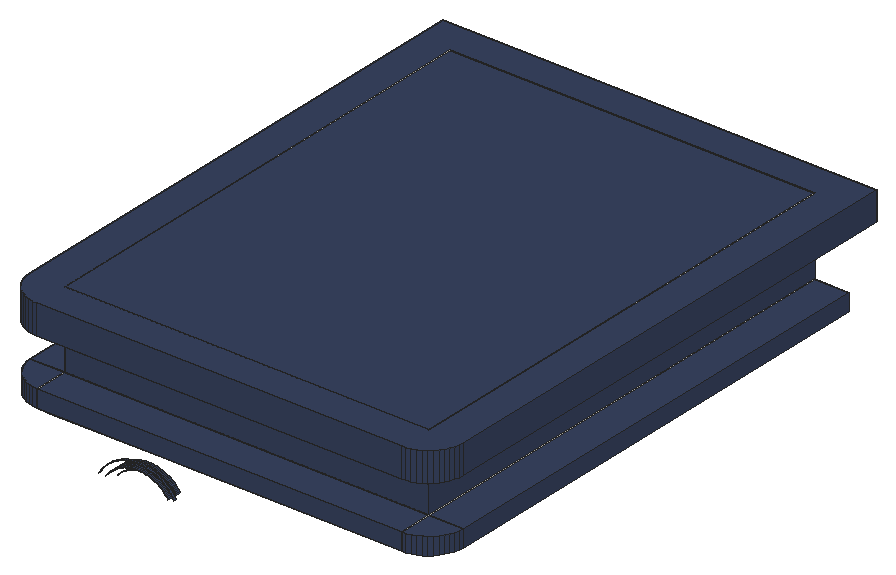
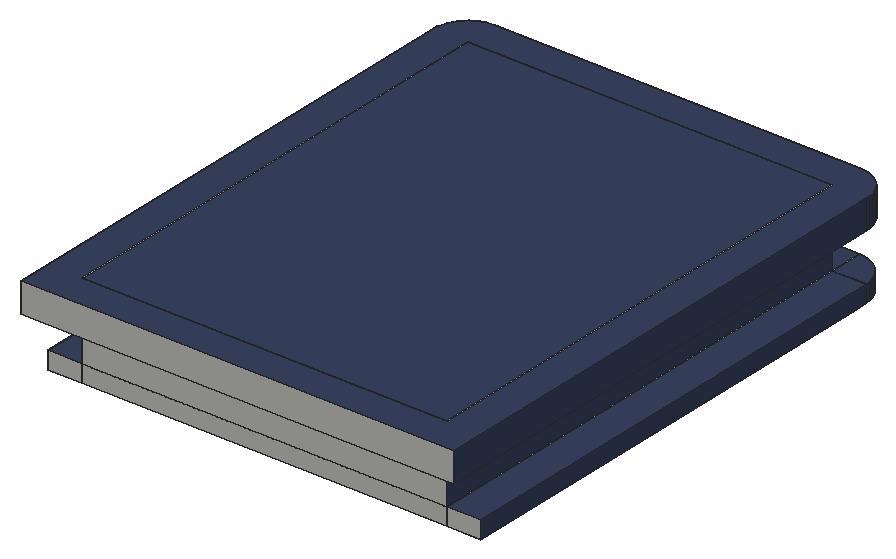
# SketchUp Ruby script. Lengths in inches.
U = 1.inch
M = Sketchup.active_model
def pt(a) = Geom::Point3d.new(a.map { |v| v * U })
def face(e, loops, mat)
  f = e.add_face(loops[0].map { |a| pt(a) })
  loops[1..].each { |l| e.add_face(l.map { |a| pt(a) }).erase! }
  f.material = f.back_material = mat if mat
  f
end
# faces: each face lists its corners as indices into pts; further lists are holes
def faces(e, pts, list, mat = nil) = list.each { |f| face(e, (f[0].is_a?(Array) ? f : [f]).map { |l| l.map { |i| pts[i] } }, mat) }
# xy, xz, yz: faces in a plane at the given z, y or x. An outline is a flat list of corners, or four numbers for a rectangle; further outlines are holes
def ring(l) = l.size == 4 ? [[l[0], l[1]], [l[2], l[1]], [l[2], l[3]], [l[0], l[3]]] : l.each_slice(2).to_a
def flat(e, list, mat, &to3) = list.each { |f| face(e, (f[0].is_a?(Array) ? f : [f]).map { |l| ring(l).map { |u, v| to3.(u, v) } }, mat) }
def xy(e, z, list, mat = nil) = flat(e, list, mat) { |x, y| [x, y, z] }
def xz(e, y, list, mat = nil) = flat(e, list, mat) { |x, z| [x, y, z] }
def yz(e, x, list, mat = nil) = flat(e, list, mat) { |y, z| [x, y, z] }
def lines(e, pts, list) = list.each { |a, b| e.add_line(pt(pts[a]), pt(pts[b])) }
# prism: a flat outline (further loops are holes) pulled along v
def prism(e, loops, v, mat = nil)
  f = face(e, loops, mat); d = Geom::Vector3d.new(v.map { |x| x * U })
  f.pushpull(f.normal.samedirection?(d) ? d.length : -d.length)
end
def box(e, o, s, mat = nil) = prism(e, [[o, [o[0] + s[0], o[1], o[2]], [o[0] + s[0], o[1] + s[1], o[2]], [o[0], o[1] + s[1], o[2]]]], [0, 0, s[2]], mat)
def at(x, y, z, deg = 0) = Geom::Transformation.translation(pt([x, y, z])) * Geom::Transformation.rotation(ORIGIN, Z_AXIS, deg.degrees)
def axes(o, x, y, z) = Geom::Transformation.new([*x, 0, *y, 0, *z, 0, *pt(o).to_a, 1])
def part(name) = M.definitions.add(name)
# library, detail: a bought-in or finely detailed component or shape, given as its bounding box
def library(name, o, s) = part(name).tap { |d| box(d.entities, o, s) }
def detail(e, o, s) = box(e.add_group.entities, o, s)
def put(e, d, t, mat = nil) = e.add_instance(d, t).tap { |i| i.material = mat if mat }
def group(e, t, mat = nil) = e.add_group.tap { |g| g.transformation = t; g.material = mat if mat }.entities
root = M.entities
M.materials.add("0360 AP 9644 Monsoon Midnight-N").color = [56, 67, 95]
M.materials.add("[Color M07]").color = [58, 58, 58]
xy(root,360,[[24,89.9375,33,98.79],[33,89.9375,117.8125,98.79],[117.8125,89.9375,126.8125,425.9375],[0,98.79,24,98.9375],[24,98.79,33,98.9375],
  [24,98.9375,33,425.9375],[126.8125,125.9375,269.3125,134.9375],[269.3125,125.9375,278.3125,134.9375],[126.8125,134.9375,269.3125,417.55],[269.3125,134.9375,278.3125,425.9375],
  [33,416.9375,117.8125,425.9375],[126.8125,417.55,269.3125,425.9375]])
xy(root,360,[[24,65.9375,20.95,66.36,17.98,67.14,15.12,68.27,12.4,69.72,9.88,71.48,7.58,73.52,5.54,75.82,3.78,78.34,2.33,81.05,1.21,83.92,0.43,86.89,0,89.9375,24,89.9375],[24,65.9375,33,89.9375],[33,65.9375,117.8125,89.9375],[117.8125,65.9375,126.8125,89.9375],[126.8125,65.9375,269.3125,89.9375],
  [269.3125,65.9375,278.3125,89.9375],[278.3125,65.9375,278.3125,89.9375,302.3125,89.9375,302.02,86.84,301.34,83.8,300.28,80.875,298.87,78.1,297.12,75.53,295.06,73.19,292.72,71.13,290.15,69.38,287.375,67.97,284.45,66.91,281.41,66.23],[0,89.9375,24,98.79],[126.8125,89.9375,269.3125,125.9375],[269.3125,89.9375,278.3125,125.9375],
  [278.3125,89.9375,302.3125,125.9375],[33,98.79,117.8125,416.9375],[0,98.9375,24,425.9375],[278.3125,125.9375,302.3125,134.9375],[278.3125,134.9375,302.3125,425.9375]],"0360 AP 9644 Monsoon Midnight-N")
xy(root,372,[[24,89.9375,278.3125,425.9375]])
xy(root,372,[[24,65.9375,24,89.9375,0,89.9375,0.43,86.89,1.21,83.92,2.33,81.05,3.78,78.34,5.54,75.82,7.58,73.52,9.88,71.48,12.4,69.72,15.12,68.27,17.98,67.14,20.95,66.36],[24,65.9375,278.3125,89.9375],[278.3125,65.9375,281.41,66.23,284.45,66.91,287.375,67.97,290.15,69.38,292.72,71.13,295.06,73.19,297.12,75.53,298.87,78.1,300.28,80.875,301.34,83.8,302.02,86.84,302.3125,89.9375,278.3125,89.9375],[0,89.9375,24,425.9375],[278.3125,89.9375,302.3125,425.9375]],"0360 AP 9644 Monsoon Midnight-N")
xy(root,405.375,[[24,89.9375,278.3125,425.9375]])
xy(root,405.375,[[[24,65.9375,20.87,66.14,17.79,66.76,14.82,67.76,12,69.15,9.39,70.9,7.03,72.97,4.96,75.33,3.22,77.9375,1.83,80.75,0.82,83.73,0.21,86.8,0,89.9375,0,449.9375,302.3125,449.9375,302.3125,89.9375,302.11,86.8,301.49,83.73,300.49,80.75,299.1,77.9375,297.35,75.33,295.28,72.97,292.92,70.9,290.3125,69.15,287.5,67.76,284.52,66.76,281.45,66.14,278.3125,65.9375],[24,89.9375,278.3125,425.9375]]],"0360 AP 9644 Monsoon Midnight-N")
xy(root,425.625,[[[24,65.9375,278.3125,65.9375,281.45,66.14,284.52,66.76,287.5,67.76,290.3125,69.15,292.92,70.9,295.28,72.97,297.35,75.33,299.1,77.9375,300.49,80.75,301.49,83.73,302.11,86.8,302.3125,89.9375,302.3125,449.9375,0,449.9375,0,89.9375,0.21,86.8,0.82,83.73,1.83,80.75,3.22,77.9375,4.96,75.33,7.03,72.97,9.39,70.9,12,69.15,14.82,67.76,17.79,66.76,20.87,66.14],[24,89.9375,278.3125,425.9375]],[24,89.9375,278.3125,425.9375]],"0360 AP 9644 Monsoon Midnight-N")
xz(root,65.9375,[[24,360,278.3125,372],[24,405.375,278.3125,425.625]],"0360 AP 9644 Monsoon Midnight-N")
xz(root,89.9375,[[0,360,24,372],[24,360,278.3125,372],[278.3125,360,302.3125,372],[24,405.375,278.3125,425.625]])
xz(root,89.9375,[[24,372,278.3125,405.375]],"0360 AP 9644 Monsoon Midnight-N")
xz(root,425.9375,[[0,360,24,372],[24,360,278.3125,372],[278.3125,360,302.3125,372],[24,372,278.3125,405.375],[24,405.375,278.3125,425.625]])
xz(root,449.9375,[[0,405.375,302.3125,425.625]])
yz(root,0,[[89.9375,360,425.9375,372],[89.9375,405.375,449.9375,425.625]],"0360 AP 9644 Monsoon Midnight-N")
yz(root,24,[[65.9375,360,89.9375,372],[89.9375,360,425.9375,372],[89.9375,405.375,425.9375,425.625]])
yz(root,24,[[89.9375,372,425.9375,405.375]],"0360 AP 9644 Monsoon Midnight-N")
yz(root,278.3125,[[65.9375,360,89.9375,372],[89.9375,360,425.9375,372],[89.9375,405.375,425.9375,425.625]])
yz(root,278.3125,[[89.9375,372,425.9375,405.375]],"0360 AP 9644 Monsoon Midnight-N")
yz(root,302.3125,[[89.9375,360,425.9375,372],[89.9375,405.375,449.9375,425.625]],"0360 AP 9644 Monsoon Midnight-N")
p = [[49.86,89.9375,319.39],[49.35,89.9375,318.51],[49.35,88.375,318.51],[49.86,88.375,319.39],[58.67,94.27,318.47],[59.18,94.27,319.04],
  [59.18,93.58,319.04],[58.67,93.58,318.47],[92.95,94.27,319.04],[93.45,94.27,318.47],[93.45,93.58,318.47],[92.95,93.58,319.04],
  [92.95,94.96,319.04],[93.45,94.96,318.47],[54.4,88.375,318.69],[54.4,93.58,318.69],[54.91,93.58,319.4],[54.91,88.375,319.4],
  [97.21,88.375,319.4],[97.21,93.58,319.4],[97.73,93.58,318.69],[97.73,88.375,318.69],[54.91,94.96,319.4],[54.4,94.96,318.69],
  [97.73,94.96,318.69],[97.21,94.96,319.4],[54.91,98.79,319.4],[54.4,98.79,318.69],[97.73,98.79,318.69],[97.21,98.79,319.4],
  [59.7,94.27,319.59],[59.7,93.58,319.59],[92.42,94.27,319.59],[92.42,93.58,319.59],[92.42,94.96,319.59],[50.4,89.9375,320.25],
  [50.4,88.375,320.25],[55.45,93.58,320.09],[55.45,88.375,320.09],[96.68,88.375,320.09],[96.68,93.58,320.09],[55.45,94.96,320.09],
  [96.68,94.96,320.09],[55.45,98.79,320.09],[96.68,98.79,320.09],[60.24,94.27,320.125],[60.24,93.58,320.125],[91.88,94.27,320.125],
  [91.88,93.58,320.125],[91.88,94.96,320.125],[101.93,89.9375,319.69],[100.8,89.9375,321.43],[100.8,88.375,321.43],[101.93,88.375,319.69],
  [56.01,93.58,320.76],[56.01,88.375,320.76],[96.12,88.375,320.76],[96.12,93.58,320.76],[56.01,94.96,320.76],[60.8,94.27,320.64],
  [60.8,93.58,320.64],[91.32,94.27,320.64],[91.32,93.58,320.64],[96.12,94.96,320.76],[91.32,94.96,320.64],[56.01,98.79,320.76],
  [96.12,98.79,320.76],[50.97,89.9375,321.09],[50.97,88.375,321.09],[61.375,94.27,321.13],[61.375,93.58,321.13],[90.75,94.27,321.13],
  [90.75,93.58,321.13],[90.75,94.96,321.13],[56.59,93.58,321.42],[56.59,88.375,321.42],[95.54,88.375,321.42],[95.54,93.58,321.42],
  [56.59,94.96,321.42],[95.54,94.96,321.42],[56.59,98.79,321.42],[95.54,98.79,321.42],[51.57,89.9375,321.91],[51.57,88.375,321.91],
  [61.97,94.27,321.61],[61.97,93.58,321.61],[90.16,94.27,321.61],[90.16,93.58,321.61],[90.16,94.96,321.61],[57.19,93.58,322.05],
  [57.19,88.375,322.05],[94.93,88.375,322.05],[94.93,93.58,322.05],[99.56,89.9375,323.08],[99.56,88.375,323.08],[57.19,94.96,322.05],
  [94.93,94.96,322.05],[57.19,98.79,322.05],[94.93,98.79,322.05],[62.57,94.27,322.07],[62.57,93.58,322.07],[89.55,94.27,322.07],
  [89.55,93.58,322.07],[89.55,94.96,322.07],[52.1875,89.9375,322.71],[52.1875,88.375,322.71],[57.81,93.58,322.67],[57.81,88.375,322.67],
  [94.31,88.375,322.67],[94.31,93.58,322.67],[57.81,94.96,322.67],[63.19,94.27,322.51],[63.19,93.58,322.51],[88.93,94.27,322.51],
  [88.93,93.58,322.51],[94.31,94.96,322.67],[88.93,94.96,322.51],[57.81,98.79,322.67],[94.31,98.79,322.67],[63.83,94.27,322.92],
  [63.83,93.58,322.92],[88.3,94.27,322.92],[88.3,93.58,322.92],[88.3,94.96,322.92],[52.84,89.9375,323.49],[52.84,88.375,323.49],
  [58.46,93.58,323.26],[58.46,88.375,323.26],[93.67,88.375,323.26],[93.67,93.58,323.26],[58.46,94.96,323.26],[93.67,94.96,323.26],
  [58.46,98.79,323.26],[93.67,98.79,323.26],[64.48,94.27,323.32],[64.48,93.58,323.32],[87.65,94.27,323.32],[87.65,93.58,323.32],
  [87.65,94.96,323.32],[98.23,89.9375,324.66],[98.23,88.375,324.66],[59.12,93.58,323.84],[59.12,88.375,323.84],[93,88.375,323.84],
  [93,93.58,323.84],[59.12,94.96,323.84],[65.14,94.27,323.6875],[65.14,93.58,323.6875],[86.99,94.27,323.6875],[86.99,93.58,323.6875],
  [93,94.96,323.84],[86.99,94.96,323.6875],[59.12,98.79,323.84],[93,98.79,323.84],[53.51,89.9375,324.25],[53.51,88.375,324.25],
  [65.8125,94.27,324.04],[65.8125,93.58,324.04],[86.3125,94.27,324.04],[86.3125,93.58,324.04],[86.3125,94.96,324.04],[59.8,93.58,324.39],
  [59.8,88.375,324.39],[92.32,88.375,324.39],[92.32,93.58,324.39],[59.8,94.96,324.39],[92.32,94.96,324.39],[59.8,98.79,324.39],
  [92.32,98.79,324.39],[66.5,94.27,324.37],[66.5,93.58,324.37],[85.63,94.27,324.37],[85.63,93.58,324.37],[85.63,94.96,324.37],
  [54.21,89.9375,324.98],[54.21,88.375,324.98],[60.5,93.58,324.91],[60.5,88.375,324.91],[91.625,88.375,324.91],[91.625,93.58,324.91],
  [60.5,94.96,324.91],[67.19,94.27,324.67],[67.19,93.58,324.67],[84.93,94.27,324.67],[84.93,93.58,324.67],[91.625,94.96,324.91],
  [84.93,94.96,324.67],[60.5,98.79,324.91],[91.625,98.79,324.91],[97.92,89.9375,324.98],[97.92,88.375,324.98],[67.9,94.27,324.95],
  [67.9,93.58,324.95],[84.23,94.27,324.95],[84.23,93.58,324.95],[84.23,94.96,324.95],[61.22,93.58,325.42],[61.22,88.375,325.42],
  [90.91,88.375,325.42],[90.91,93.58,325.42],[61.22,94.96,325.42],[90.91,94.96,325.42],[61.22,98.79,325.42],[90.91,98.79,325.42],
  [54.93,89.9375,325.7],[54.93,88.375,325.7],[97.2,89.9375,325.7],[97.2,88.375,325.7],[68.61,94.27,325.21],[68.61,93.58,325.21],
  [83.52,94.27,325.21],[83.52,93.58,325.21],[83.52,94.96,325.21],[69.33,94.27,325.45],[69.33,93.58,325.45],[82.79,94.27,325.45],
  [82.79,93.58,325.45],[82.79,94.96,325.45],[61.95,93.58,325.9],[61.95,88.375,325.9],[90.17,88.375,325.9],[90.17,93.58,325.9],
  [61.95,94.96,325.9],[70.06,94.27,325.66],[70.06,93.58,325.66],[82.06,94.27,325.66],[82.06,93.58,325.66],[90.17,94.96,325.9],
  [82.06,94.96,325.66],[61.95,98.79,325.9],[90.17,98.79,325.9],[55.67,89.9375,326.38],[55.67,88.375,326.38],[96.45,89.9375,326.38],
  [96.45,88.375,326.38],[70.8,94.27,325.85],[70.8,93.58,325.85],[81.33,94.27,325.85],[81.33,93.58,325.85],[81.33,94.96,325.85],
  [71.54,94.27,326.01],[71.54,93.58,326.01],[80.59,94.27,326.01],[80.59,93.58,326.01],[80.59,94.96,326.01],[62.7,93.58,326.35],
  [62.7,88.375,326.35],[89.43,88.375,326.35],[89.43,93.58,326.35],[62.7,94.96,326.35],[89.43,94.96,326.35],[62.7,98.79,326.35],
  [89.43,98.79,326.35],[72.28,94.27,326.15],[72.28,93.58,326.15],[79.84,94.27,326.15],[79.84,93.58,326.15],[79.84,94.96,326.15],
  [73.03,94.27,326.26],[73.03,93.58,326.26],[79.09,94.27,326.26],[79.09,93.58,326.26],[79.09,94.96,326.26],[73.03,94.96,326.26],
  [73.79,94.96,326.35],[73.79,93.58,326.35],[74.55,94.96,326.41],[74.55,93.58,326.41],[77.58,94.27,326.41],[78.34,94.27,326.35],
  [78.34,93.58,326.35],[77.58,93.58,326.41],[77.58,94.96,326.41],[78.34,94.96,326.35],[56.44,89.9375,327.05],[56.44,88.375,327.05],
  [63.46,93.58,326.78],[63.46,88.375,326.78],[88.66,88.375,326.78],[88.66,93.58,326.78],[95.68,89.9375,327.05],[95.68,88.375,327.05],
  [63.46,94.96,326.78],[75.3,94.96,326.45],[75.3,93.58,326.45],[76.0625,94.96,326.46],[76.0625,94.27,326.46],[76.0625,93.58,326.46],
  [76.82,94.27,326.45],[76.82,93.58,326.45],[88.66,94.96,326.78],[76.82,94.96,326.45],[63.46,98.79,326.78],[88.66,98.79,326.78],
  [64.24,93.58,327.18],[64.24,88.375,327.18],[87.89,88.375,327.18],[87.89,93.58,327.18],[64.24,94.96,327.18],[87.89,94.96,327.18],
  [64.24,98.79,327.18],[87.89,98.79,327.18],[57.23,89.9375,327.68],[57.23,88.375,327.68],[94.89,89.9375,327.68],[94.89,88.375,327.68],
  [65.03,93.58,327.5625],[65.03,88.375,327.5625],[87.1,88.375,327.5625],[87.1,93.58,327.5625],[65.03,94.96,327.5625],[87.1,94.96,327.5625],
  [65.03,98.79,327.5625],[87.1,98.79,327.5625],[65.83,93.58,327.92],[65.83,88.375,327.92],[86.3,88.375,327.92],[86.3,93.58,327.92],
  [65.83,94.96,327.92],[86.3,94.96,327.92],[65.83,98.79,327.92],[86.3,98.79,327.92],[58.04,89.9375,328.29],[58.04,88.375,328.29],
  [94.08,89.9375,328.29],[94.08,88.375,328.29],[66.64,93.58,328.24],[66.64,88.375,328.24],[85.48,88.375,328.24],[85.48,93.58,328.24],
  [66.64,94.96,328.24],[85.48,94.96,328.24],[66.64,98.79,328.24],[85.48,98.79,328.24],[67.47,93.58,328.54],[67.47,88.375,328.54],
  [84.66,88.375,328.54],[84.66,93.58,328.54],[67.47,94.96,328.54],[84.66,94.96,328.54],[67.47,98.79,328.54],[84.66,98.79,328.54],
  [58.87,89.9375,328.875],[58.87,88.375,328.875],[93.25,89.9375,328.875],[93.25,88.375,328.875],[68.3,93.58,328.81],[68.3,88.375,328.81],
  [83.83,88.375,328.81],[83.83,93.58,328.81],[68.3,94.96,328.81],[83.83,94.96,328.81],[68.3,98.79,328.81],[83.83,98.79,328.81],
  [69.14,93.58,329.05],[69.14,88.375,329.05],[82.99,88.375,329.05],[82.99,93.58,329.05],[69.14,94.96,329.05],[82.99,94.96,329.05],
  [69.14,98.79,329.05],[82.99,98.79,329.05],[59.72,89.9375,329.43],[59.72,88.375,329.43],[92.41,89.9375,329.43],[92.41,88.375,329.43],
  [69.99,93.58,329.27],[69.99,88.375,329.27],[82.14,88.375,329.27],[82.14,93.58,329.27],[69.99,94.96,329.27],[82.14,94.96,329.27],
  [69.99,98.79,329.27],[82.14,98.79,329.27],[70.84,93.58,329.46],[70.84,88.375,329.46],[81.28,88.375,329.46],[81.28,93.58,329.46],
  [70.84,94.96,329.46],[81.28,94.96,329.46],[70.84,98.79,329.46],[81.28,98.79,329.46],[60.59,89.9375,329.96],[60.59,88.375,329.96],
  [91.54,89.9375,329.96],[91.54,88.375,329.96],[71.7,93.58,329.61],[71.7,88.375,329.61],[80.42,88.375,329.61],[80.42,93.58,329.61],
  [71.7,94.96,329.61],[80.42,94.96,329.61],[71.7,98.79,329.61],[80.42,98.79,329.61],[72.57,93.58,329.74],[72.57,88.375,329.74],
  [79.55,88.375,329.74],[79.55,93.58,329.74],[72.57,94.96,329.74],[79.55,94.96,329.74],[72.57,98.79,329.74],[79.55,98.79,329.74],
  [73.44,93.58,329.85],[73.44,88.375,329.85],[78.69,88.375,329.85],[78.69,93.58,329.85],[73.44,94.96,329.85],[78.69,94.96,329.85],
  [73.44,98.79,329.85],[78.69,98.79,329.85],[74.3125,93.58,329.92],[74.3125,88.375,329.92],[77.8125,88.375,329.92],[77.8125,93.58,329.92],
  [74.3125,94.96,329.92],[77.8125,94.96,329.92],[74.3125,98.79,329.92],[77.8125,98.79,329.92],[75.1875,93.58,329.96],[75.1875,88.375,329.96],
  [76.9375,88.375,329.96],[76.9375,93.58,329.96],[75.1875,94.96,329.96],[76.9375,94.96,329.96],[75.1875,98.79,329.96],[76.9375,98.79,329.96],
  [61.47,89.9375,330.46],[61.47,88.375,330.46],[76.0625,93.58,329.98],[76.0625,88.375,329.98],[90.66,89.9375,330.46],[90.66,88.375,330.46],
  [76.0625,94.96,329.98],[76.0625,98.79,329.98],[62.37,89.9375,330.92],[62.37,88.375,330.92],[89.76,89.9375,330.92],[89.76,88.375,330.92],
  [63.28,89.9375,331.36],[63.28,88.375,331.36],[88.84,89.9375,331.36],[88.84,88.375,331.36],[64.21,89.9375,331.77],[64.21,88.375,331.77],
  [87.91,89.9375,331.77],[87.91,88.375,331.77],[65.15,89.9375,332.15],[65.15,88.375,332.15],[86.97,89.9375,332.15],[86.97,88.375,332.15],
  [66.11,89.9375,332.49],[66.11,88.375,332.49],[86.02,89.9375,332.49],[86.02,88.375,332.49],[67.07,89.9375,332.81],[67.07,88.375,332.81],
  [85.06,89.9375,332.81],[85.06,88.375,332.81],[68.04,89.9375,333.09],[68.04,88.375,333.09],[84.08,89.9375,333.09],[84.08,88.375,333.09],
  [69.03,89.9375,333.34],[69.03,88.375,333.34],[83.1,89.9375,333.34],[83.1,88.375,333.34],[70.02,89.9375,333.55],[70.02,88.375,333.55],
  [82.11,89.9375,333.55],[82.11,88.375,333.55],[71.02,89.9375,333.74],[71.02,88.375,333.74],[81.11,89.9375,333.74],[81.11,88.375,333.74],
  [72.02,89.9375,333.89],[72.02,88.375,333.89],[80.11,89.9375,333.89],[80.11,88.375,333.89],[73.03,89.9375,334.01],[73.03,88.375,334.01],
  [79.1,89.9375,334.01],[79.1,88.375,334.01],[74.04,89.9375,334.09],[74.04,88.375,334.09],[78.09,89.9375,334.09],[78.09,88.375,334.09],
  [75.05,89.9375,334.14],[75.05,88.375,334.14],[76.0625,89.9375,334.16],[76.0625,88.375,334.16],[77.08,89.9375,334.14],[77.08,88.375,334.14],
  [24,65.9375,372],[20.95,66.36,372],[20.95,66.36,360],[24,65.9375,360],[281.41,66.23,372],[278.3125,65.9375,372],
  [278.3125,65.9375,360],[281.41,66.23,360],[284.45,66.91,372],[284.45,66.91,360],[17.98,67.14,372],[17.98,67.14,360],
  [287.375,67.97,372],[287.375,67.97,360],[15.12,68.27,372],[15.12,68.27,360],[290.15,69.38,372],[290.15,69.38,360],
  [12.4,69.72,372],[12.4,69.72,360],[292.72,71.13,372],[292.72,71.13,360],[9.88,71.48,372],[9.88,71.48,360],
  [295.06,73.19,372],[295.06,73.19,360],[7.58,73.52,372],[7.58,73.52,360],[297.12,75.53,372],[297.12,75.53,360],
  [5.54,75.82,372],[5.54,75.82,360],[298.87,78.1,372],[298.87,78.1,360],[3.78,78.34,372],[3.78,78.34,360],
  [300.28,80.875,372],[300.28,80.875,360],[2.33,81.05,372],[2.33,81.05,360],[301.34,83.8,372],[301.34,83.8,360],
  [1.21,83.92,372],[1.21,83.92,360],[302.02,86.84,372],[302.02,86.84,360],[0.43,86.89,372],[0.43,86.89,360],
  [302.3125,89.9375,372],[302.3125,89.9375,360],[0,89.9375,372],[0,89.9375,360],[24,65.9375,425.625],[20.87,66.14,425.625],
  [20.87,66.14,405.375],[24,65.9375,405.375],[281.45,66.14,425.625],[278.3125,65.9375,425.625],[278.3125,65.9375,405.375],[281.45,66.14,405.375],
  [17.79,66.76,425.625],[17.79,66.76,405.375],[284.52,66.76,425.625],[284.52,66.76,405.375],[14.82,67.76,425.625],[14.82,67.76,405.375],
  [287.5,67.76,425.625],[287.5,67.76,405.375],[12,69.15,425.625],[12,69.15,405.375],[290.3125,69.15,425.625],[290.3125,69.15,405.375],
  [9.39,70.9,425.625],[9.39,70.9,405.375],[292.92,70.9,425.625],[292.92,70.9,405.375],[7.03,72.97,425.625],[7.03,72.97,405.375],
  [295.28,72.97,425.625],[295.28,72.97,405.375],[4.96,75.33,425.625],[4.96,75.33,405.375],[297.35,75.33,425.625],[297.35,75.33,405.375],
  [3.22,77.9375,425.625],[3.22,77.9375,405.375],[299.1,77.9375,425.625],[299.1,77.9375,405.375],[1.83,80.75,425.625],[1.83,80.75,405.375],
  [300.49,80.75,425.625],[300.49,80.75,405.375],[0.82,83.73,425.625],[0.82,83.73,405.375],[301.49,83.73,425.625],[301.49,83.73,405.375],
  [0.21,86.8,425.625],[0.21,86.8,405.375],[302.11,86.8,425.625],[302.11,86.8,405.375],[0,89.9375,425.625],[0,89.9375,405.375],
  [302.3125,89.9375,425.625],[302.3125,89.9375,405.375],[72.28,94.96,326.15],[71.54,94.96,326.01],[70.8,94.96,325.85],[70.06,94.96,325.66],
  [69.33,94.96,325.45],[68.61,94.96,325.21],[67.9,94.96,324.95],[67.19,94.96,324.67],[66.5,94.96,324.37],[65.8125,94.96,324.04],
  [65.14,94.96,323.6875],[64.48,94.96,323.32],[63.83,94.96,322.92],[63.19,94.96,322.51],[62.57,94.96,322.07],[61.97,94.96,321.61],
  [61.375,94.96,321.13],[60.8,94.96,320.64],[60.24,94.96,320.125],[59.7,94.96,319.59],[59.18,94.96,319.04],[58.67,94.96,318.47]]
faces(root,p,[[0,1,2,3],[14,15,16,17],[18,19,20,21],[26,22,23,27],[28,24,25,29],[35,0,3,36],[17,16,37,38],[39,40,19,18],
  [43,41,22,26],[29,25,42,44],[50,51,52,53],[38,37,54,55],[56,57,40,39],[65,58,41,43],[44,42,63,66],[67,35,36,68],
  [55,54,74,75],[76,77,57,56],[80,78,58,65],[66,63,79,81],[82,67,68,83],[75,74,89,90],[91,92,77,76],[51,93,94,52],
  [97,95,78,80],[81,79,96,98],[104,82,83,105],[90,89,106,107],[108,109,92,91],[117,110,95,97],[98,96,115,118],[124,104,105,125],
  [107,106,126,127],[128,129,109,108],[132,130,110,117],[118,115,131,133],[93,139,140,94],[127,126,141,142],[143,144,129,128],[152,145,130,132],
  [133,131,150,153],[154,124,125,155],[142,141,161,162],[163,164,144,143],[167,165,145,152],[153,150,166,168],[174,154,155,175],[162,161,176,177],
  [178,179,164,163],[187,180,165,167],[168,166,185,188],[139,189,190,140],[177,176,196,197],[198,199,179,178],[202,200,180,187],[188,185,201,203],
  [204,174,175,205],[189,206,207,190],[197,196,218,219],[220,221,199,198],[229,222,200,202],[203,201,227,230],[231,204,205,232],[206,233,234,207],
  [219,218,245,246],[247,248,221,220],[251,249,222,229],[230,227,250,252],[274,231,232,275],[246,245,276,277],[278,279,248,247],[233,280,281,234],
  [292,282,249,251],[252,250,290,293],[277,276,294,295],[296,297,279,278],[300,298,282,292],[293,290,299,301],[302,274,275,303],[280,304,305,281],
  [295,294,306,307],[308,309,297,296],[312,310,298,300],[301,299,311,313],[307,306,314,315],[316,317,309,308],[320,318,310,312],[313,311,319,321],
  [322,302,303,323],[304,324,325,305],[315,314,326,327],[328,329,317,316],[332,330,318,320],[321,319,331,333],[327,326,334,335],[336,337,329,328],
  [340,338,330,332],[333,331,339,341],[342,322,323,343],[324,344,345,325],[335,334,346,347],[348,349,337,336],[352,350,338,340],[341,339,351,353],
  [347,346,354,355],[356,357,349,348],[360,358,350,352],[353,351,359,361],[362,342,343,363],[344,364,365,345],[355,354,366,367],[368,369,357,356],
  [372,370,358,360],[361,359,371,373],[367,366,374,375],[376,377,369,368],[380,378,370,372],[373,371,379,381],[382,362,363,383],[364,384,385,365],
  [375,374,386,387],[388,389,377,376],[392,390,378,380],[381,379,391,393],[387,386,394,395],[396,397,389,388],[400,398,390,392],[393,391,399,401],
  [395,394,402,403],[404,405,397,396],[408,406,398,400],[401,399,407,409],[403,402,410,411],[412,413,405,404],[416,414,406,408],[409,407,415,417],
  [411,410,418,419],[420,421,413,412],[424,422,414,416],[417,415,423,425],[426,382,383,427],[419,418,428,429],[429,428,421,420],[384,430,431,385],
  [433,432,422,424],[425,423,432,433],[434,426,427,435],[430,436,437,431],[438,434,435,439],[436,440,441,437],[442,438,439,443],[440,444,445,441],
  [446,442,443,447],[444,448,449,445],[450,446,447,451],[448,452,453,449],[454,450,451,455],[452,456,457,453],[458,454,455,459],[456,460,461,457],
  [462,458,459,463],[460,464,465,461],[466,462,463,467],[464,468,469,465],[470,466,467,471],[468,472,473,469],[474,470,471,475],[472,476,477,473],
  [478,474,475,479],[476,480,481,477],[482,478,479,483],[480,484,485,481],[486,482,483,487],[488,486,487,489],[490,488,489,491],[484,490,491,485],
  [492,493,494,495],[496,497,498,499],[500,496,499,501],[493,502,503,494],[504,500,501,505],[502,506,507,503],[508,504,505,509],[506,510,511,507],
  [512,508,509,513],[510,514,515,511],[516,512,513,517],[514,518,519,515],[520,516,517,521],[518,522,523,519],[524,520,521,525],[522,526,527,523],
  [528,524,525,529],[526,530,531,527],[532,528,529,533],[530,534,535,531],[536,532,533,537],[534,538,539,535],[540,536,537,541],[538,542,543,539],
  [544,545,546,547],[548,549,550,551],[545,552,553,546],[554,548,551,555],[552,556,557,553],[558,554,555,559],[556,560,561,557],[562,558,559,563],
  [560,564,565,561],[566,562,563,567],[564,568,569,565],[570,566,567,571],[568,572,573,569],[574,570,571,575],[572,576,577,573],[578,574,575,579],
  [576,580,581,577],[582,578,579,583],[580,584,585,581],[586,582,583,587],[584,588,589,585],[590,586,587,591],[588,592,593,589],[594,590,591,595]],"0360 AP 9644 Monsoon Midnight-N")
faces(root,p,[[4,5,6,7],[8,9,10,11],[22,23,15,16],[24,25,19,20],[5,30,31,6],[32,8,11,33],[41,22,16,37],[25,42,40,19],
  [30,45,46,31],[47,32,33,48],[58,41,37,54],[45,59,60,46],[61,47,48,62],[42,63,57,40],[59,69,70,60],[71,61,62,72],
  [78,58,54,74],[63,79,77,57],[69,84,85,70],[86,71,72,87],[95,78,74,89],[79,96,92,77],[84,99,100,85],[101,86,87,102],
  [110,95,89,106],[99,111,112,100],[113,101,102,114],[96,115,109,92],[111,119,120,112],[121,113,114,122],[130,110,106,126],[115,131,129,109],
  [119,134,135,120],[136,121,122,137],[145,130,126,141],[134,146,147,135],[148,136,137,149],[131,150,144,129],[146,156,157,147],[158,148,149,159],
  [165,145,141,161],[150,166,164,144],[156,169,170,157],[171,158,159,172],[180,165,161,176],[169,181,182,170],[183,171,172,184],[166,185,179,164],
  [181,191,192,182],[193,183,184,194],[200,180,176,196],[185,201,199,179],[191,208,209,192],[210,193,194,211],[208,213,214,209],[215,210,211,216],
  [222,200,196,218],[213,223,224,214],[225,215,216,226],[201,227,221,199],[223,235,236,224],[237,225,226,238],[235,240,241,236],[242,237,238,243],
  [249,222,218,245],[227,250,248,221],[240,253,254,241],[255,242,243,256],[253,258,259,254],[260,255,256,261],[268,269,270,271],[269,260,261,270],
  [282,249,245,276],[286,288,289,287],[288,268,271,289],[250,290,279,248],[298,282,276,294],[290,299,297,279],[310,298,294,306],[299,311,309,297],
  [318,310,306,314],[311,319,317,309],[330,318,314,326],[319,331,329,317],[338,330,326,334],[331,339,337,329],[350,338,334,346],[339,351,349,337],
  [358,350,346,354],[351,359,357,349],[370,358,354,366],[359,371,369,357],[378,370,366,374],[371,379,377,369],[390,378,374,386],[379,391,389,377],
  [398,390,386,394],[391,399,397,389],[406,398,394,402],[399,407,405,397],[414,406,402,410],[407,415,413,405],[422,414,410,418],[415,423,421,413],
  [432,422,418,428],[423,432,428,421]],"[Color M07]")
faces(root,p,[[12,13,9,8],[34,12,8,32],[49,34,32,47],[64,49,47,61],[73,64,61,71],[88,73,71,86],[103,88,86,101],[116,103,101,113],
  [123,116,113,121],[138,123,121,136],[151,138,136,148],[160,151,148,158],[173,160,158,171],[186,173,171,183],[195,186,183,193],[212,195,193,210],
  [217,212,210,215],[228,217,215,225],[239,228,225,237],[244,239,237,242],[257,244,242,255],[262,257,255,260],[263,264,265,259,258],[264,266,267,265],
  [272,273,269,268],[273,262,260,269],[266,283,284,267],[283,285,286,287,284],[285,291,288,286],[291,272,268,288]])
lines(root,p,[[596,253],[597,240],[598,235],[599,223],[600,213],[601,208],[602,191],[603,181],[604,169],[605,156],[606,146],[607,134],
  [608,119],[609,111],[610,99],[611,84],[612,69],[613,59],[614,45],[615,30],[616,5],[617,4]])
